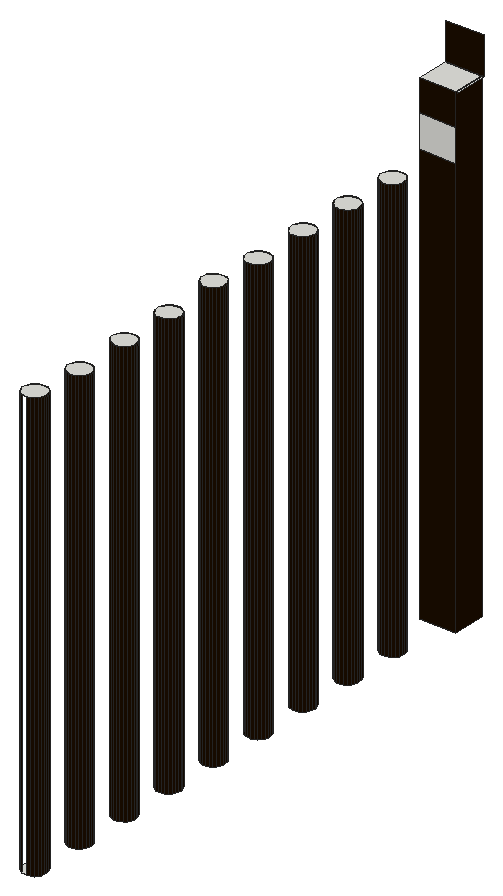
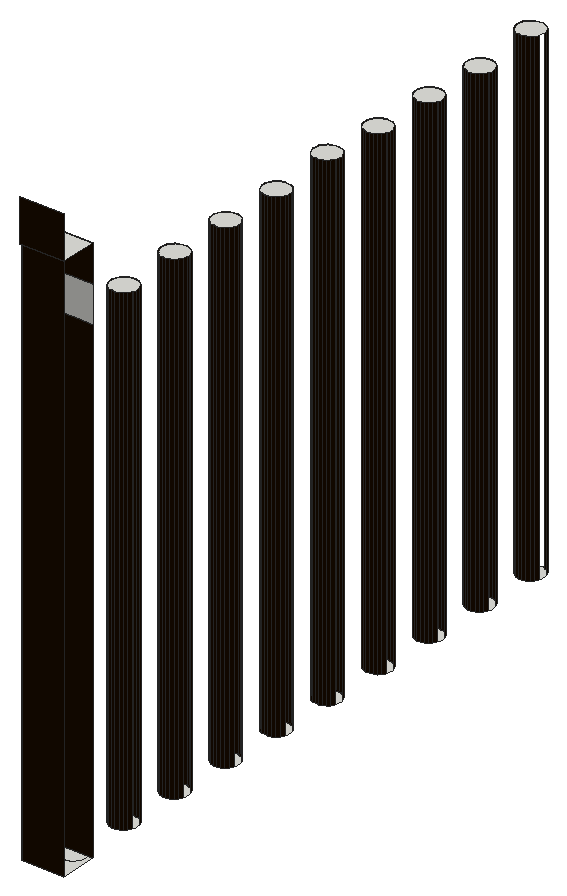
# SketchUp Ruby script. Lengths in inches.
U = 1.inch
M = Sketchup.active_model
def pt(a) = Geom::Point3d.new(a.map { |v| v * U })
def face(e, loops, mat)
  f = e.add_face(loops[0].map { |a| pt(a) })
  loops[1..].each { |l| e.add_face(l.map { |a| pt(a) }).erase! }
  f.material = f.back_material = mat if mat
  f
end
# faces: each face lists its corners as indices into pts; further lists are holes
def faces(e, pts, list, mat = nil) = list.each { |f| face(e, (f[0].is_a?(Array) ? f : [f]).map { |l| l.map { |i| pts[i] } }, mat) }
# xy, xz, yz: faces in a plane at the given z, y or x. An outline is a flat list of corners, or four numbers for a rectangle; further outlines are holes
def ring(l) = l.size == 4 ? [[l[0], l[1]], [l[2], l[1]], [l[2], l[3]], [l[0], l[3]]] : l.each_slice(2).to_a
def flat(e, list, mat, &to3) = list.each { |f| face(e, (f[0].is_a?(Array) ? f : [f]).map { |l| ring(l).map { |u, v| to3.(u, v) } }, mat) }
def xy(e, z, list, mat = nil) = flat(e, list, mat) { |x, y| [x, y, z] }
def xz(e, y, list, mat = nil) = flat(e, list, mat) { |x, z| [x, y, z] }
def yz(e, x, list, mat = nil) = flat(e, list, mat) { |y, z| [x, y, z] }
def lines(e, pts, list) = list.each { |a, b| e.add_line(pt(pts[a]), pt(pts[b])) }
# prism: a flat outline (further loops are holes) pulled along v
def prism(e, loops, v, mat = nil)
  f = face(e, loops, mat); d = Geom::Vector3d.new(v.map { |x| x * U })
  f.pushpull(f.normal.samedirection?(d) ? d.length : -d.length)
end
def box(e, o, s, mat = nil) = prism(e, [[o, [o[0] + s[0], o[1], o[2]], [o[0] + s[0], o[1] + s[1], o[2]], [o[0], o[1] + s[1], o[2]]]], [0, 0, s[2]], mat)
def at(x, y, z, deg = 0) = Geom::Transformation.translation(pt([x, y, z])) * Geom::Transformation.rotation(ORIGIN, Z_AXIS, deg.degrees)
def axes(o, x, y, z) = Geom::Transformation.new([*x, 0, *y, 0, *z, 0, *pt(o).to_a, 1])
def part(name) = M.definitions.add(name)
# library, detail: a bought-in or finely detailed component or shape, given as its bounding box
def library(name, o, s) = part(name).tap { |d| box(d.entities, o, s) }
def detail(e, o, s) = box(e.add_group.entities, o, s)
def put(e, d, t, mat = nil) = e.add_instance(d, t).tap { |i| i.material = mat if mat }
def group(e, t, mat = nil) = e.add_group.tap { |g| g.transformation = t; g.material = mat if mat }.entities
root = M.entities
M.materials.add("[Metal Seamed]1").color = [28, 14, 0]
xy(root,618.25,[[363.55,258.66,363.21,258.75,362.92,258.92,362.67,259.16,362.5,259.46,362.41,259.79,362.41,260.13,362.5,260.46,362.67,260.76,362.91,261,363.2,261.17,363.54,261.26,363.88,261.26,364.21,261.18,364.51,261.01,364.75,260.76,364.92,260.47,365.01,260.14,365.01,259.8,364.93,259.46,364.76,259.17,364.51,258.92,364.22,258.75,363.89,258.66],[363.55,265.1,363.21,265.19,362.92,265.36,362.67,265.6,362.5,265.89,362.41,266.22,362.41,266.57,362.5,266.9,362.67,267.19,362.91,267.4375,363.2,267.61,363.54,267.7,363.88,267.7,364.21,267.61,364.51,267.44,364.75,267.2,364.92,266.91,365.01,266.58,365.01,266.23,364.93,265.9,364.76,265.6,364.51,265.36,364.22,265.1875,363.89,265.1],[363.55,271.54,363.21,271.62,362.92,271.79,362.67,272.03,362.5,272.33,362.41,272.66,362.41,273,362.5,273.33,362.67,273.63,362.91,273.875,363.2,274.05,363.54,274.14,363.88,274.14,364.21,274.05,364.51,273.88,364.75,273.64,364.92,273.34,365.01,273.01,365.01,272.67,364.93,272.34,364.76,272.04,364.51,271.8,364.22,271.625,363.89,271.54],[363.55,277.97,363.21,278.06,362.92,278.23,362.67,278.47,362.5,278.77,362.41,279.1,362.41,279.44,362.5,279.77,362.67,280.07,362.91,280.3125,363.2,280.49,363.54,280.58,363.88,280.58,364.21,280.49,364.51,280.32,364.75,280.08,364.92,279.78,365.01,279.45,365.01,279.11,364.93,278.78,364.76,278.48,364.51,278.24,364.22,278.0625,363.89,277.97],[363.55,284.41,363.21,284.5,362.92,284.67,362.67,284.91,362.5,285.21,362.41,285.54,362.41,285.88,362.5,286.21,362.67,286.51,362.91,286.75,363.2,286.92,363.54,287.01,363.88,287.01,364.21,286.93,364.51,286.76,364.75,286.51,364.92,286.22,365.01,285.89,365.01,285.55,364.93,285.21,364.76,284.92,364.51,284.67,364.22,284.5,363.89,284.41],
  [363.55,290.85,363.21,290.94,362.92,291.11,362.67,291.35,362.5,291.64,362.41,291.97,362.41,292.32,362.5,292.65,362.67,292.94,362.91,293.1875,363.2,293.36,363.54,293.45,363.88,293.45,364.21,293.36,364.51,293.19,364.75,292.95,364.92,292.66,365.01,292.33,365.01,291.98,364.93,291.65,364.76,291.35,364.51,291.11,364.22,290.9375,363.89,290.85],[363.55,297.29,363.21,297.37,362.92,297.54,362.67,297.78,362.5,298.08,362.41,298.41,362.41,298.75,362.5,299.08,362.67,299.38,362.91,299.625,363.2,299.8,363.54,299.89,363.88,299.89,364.21,299.8,364.51,299.63,364.75,299.39,364.92,299.09,365.01,298.76,365.01,298.42,364.93,298.09,364.76,297.79,364.51,297.55,364.22,297.375,363.89,297.29],[363.55,303.72,363.21,303.81,362.92,303.98,362.67,304.22,362.5,304.52,362.41,304.85,362.41,305.19,362.5,305.52,362.67,305.82,362.91,306.0625,363.2,306.24,363.54,306.33,363.88,306.33,364.21,306.24,364.51,306.07,364.75,305.83,364.92,305.53,365.01,305.2,365.01,304.86,364.93,304.53,364.76,304.23,364.51,303.99,364.22,303.8125,363.89,303.72],[363.55,310.16,363.21,310.25,362.92,310.42,362.67,310.66,362.5,310.96,362.41,311.29,362.41,311.63,362.5,311.96,362.67,312.26,362.91,312.5,363.2,312.67,363.54,312.76,363.88,312.76,364.21,312.68,364.51,312.51,364.75,312.26,364.92,311.97,365.01,311.64,365.01,311.3,364.93,310.96,364.76,310.67,364.51,310.42,364.22,310.25,363.89,310.16],[361.98,317.52,361.98,321.28,366.15,321.28,366.15,317.52,364.96,317.52,365.01,317.73,365.01,318.08,364.92,318.41,364.75,318.7,364.51,318.94,364.21,319.11,363.88,319.2,363.54,319.2,363.2,319.11,362.91,318.9375,362.67,318.69,362.5,318.4,362.41,318.07,362.41,317.72,362.47,317.52],
  [362.47,317.52,364.96,317.52,365.01,317.73,365.01,318.08,364.92,318.41,364.75,318.7,364.51,318.94,364.21,319.11,363.88,319.2,363.54,319.2,363.2,319.11,362.91,318.9375,362.67,318.69,362.5,318.4,362.41,318.07,362.41,317.72]])
xy(root,667,[[363.55,310.16,363.89,310.16,364.22,310.25,364.51,310.42,364.76,310.67,364.93,310.96,365.01,311.3,365.01,311.64,364.92,311.97,364.75,312.26,364.51,312.51,364.21,312.68,363.88,312.76,363.54,312.76,363.2,312.67,362.91,312.5,362.67,312.26,362.5,311.96,362.41,311.63,362.41,311.29,362.5,310.96,362.67,310.66,362.92,310.42,363.21,310.25]])
xy(root,667.0625,[[363.55,265.1,363.89,265.1,364.22,265.1875,364.51,265.36,364.76,265.6,364.93,265.9,365.01,266.23,365.01,266.58,364.92,266.91,364.75,267.2,364.51,267.44,364.21,267.61,363.88,267.7,363.54,267.7,363.2,267.61,362.91,267.4375,362.67,267.19,362.5,266.9,362.41,266.57,362.41,266.22,362.5,265.89,362.67,265.6,362.92,265.36,363.21,265.19]])
xy(root,667.1875,[[363.55,290.85,363.89,290.85,364.22,290.9375,364.51,291.11,364.76,291.35,364.93,291.65,365.01,291.98,365.01,292.33,364.92,292.66,364.75,292.95,364.51,293.19,364.21,293.36,363.88,293.45,363.54,293.45,363.2,293.36,362.91,293.1875,362.67,292.94,362.5,292.65,362.41,292.32,362.41,291.97,362.5,291.64,362.67,291.35,362.92,291.11,363.21,290.94],[363.55,303.72,363.89,303.72,364.22,303.8125,364.51,303.99,364.76,304.23,364.93,304.53,365.01,304.86,365.01,305.2,364.92,305.53,364.75,305.83,364.51,306.07,364.21,306.24,363.88,306.33,363.54,306.33,363.2,306.24,362.91,306.0625,362.67,305.82,362.5,305.52,362.41,305.19,362.41,304.85,362.5,304.52,362.67,304.22,362.92,303.98,363.21,303.81]])
xy(root,667.25,[[363.55,271.54,363.89,271.54,364.22,271.625,364.51,271.8,364.76,272.04,364.93,272.34,365.01,272.67,365.01,273.01,364.92,273.34,364.75,273.64,364.51,273.88,364.21,274.05,363.88,274.14,363.54,274.14,363.2,274.05,362.91,273.875,362.67,273.63,362.5,273.33,362.41,273,362.41,272.66,362.5,272.33,362.67,272.03,362.92,271.79,363.21,271.62],[363.55,277.97,363.89,277.97,364.22,278.0625,364.51,278.24,364.76,278.48,364.93,278.78,365.01,279.11,365.01,279.45,364.92,279.78,364.75,280.08,364.51,280.32,364.21,280.49,363.88,280.58,363.54,280.58,363.2,280.49,362.91,280.3125,362.67,280.07,362.5,279.77,362.41,279.44,362.41,279.1,362.5,278.77,362.67,278.47,362.92,278.23,363.21,278.06],[363.55,297.29,363.89,297.29,364.22,297.375,364.51,297.55,364.76,297.79,364.93,298.09,365.01,298.42,365.01,298.76,364.92,299.09,364.75,299.39,364.51,299.63,364.21,299.8,363.88,299.89,363.54,299.89,363.2,299.8,362.91,299.625,362.67,299.38,362.5,299.08,362.41,298.75,362.41,298.41,362.5,298.08,362.67,297.78,362.92,297.54,363.21,297.37]])
xy(root,667.625,[[363.55,258.66,363.89,258.66,364.22,258.75,364.51,258.92,364.76,259.17,364.93,259.46,365.01,259.8,365.01,260.14,364.92,260.47,364.75,260.76,364.51,261.01,364.21,261.18,363.88,261.26,363.54,261.26,363.2,261.17,362.91,261,362.67,260.76,362.5,260.46,362.41,260.13,362.41,259.79,362.5,259.46,362.67,259.16,362.92,258.92,363.21,258.75]])
xy(root,667.6875,[[363.55,284.41,363.89,284.41,364.22,284.5,364.51,284.67,364.76,284.92,364.93,285.21,365.01,285.55,365.01,285.89,364.92,286.22,364.75,286.51,364.51,286.76,364.21,286.93,363.88,287.01,363.54,287.01,363.2,286.92,362.91,286.75,362.67,286.51,362.5,286.21,362.41,285.88,362.41,285.54,362.5,285.21,362.67,284.91,362.92,284.67,363.21,284.5]])
xy(root,674.05,[[361.98,317.52,366.15,321.28],[366.15,317.52,366.34,321.28]])
xz(root,261.26,[[363.54,618.25,363.88,667.625]],"[Metal Seamed]1")
xz(root,265.1,[[363.55,618.25,363.89,667.0625]],"[Metal Seamed]1")
xz(root,267.7,[[363.54,618.25,363.88,667.0625]],"[Metal Seamed]1")
xz(root,271.54,[[363.55,618.25,363.89,667.25]],"[Metal Seamed]1")
xz(root,274.14,[[363.54,618.25,363.88,667.25]],"[Metal Seamed]1")
xz(root,277.97,[[363.55,618.25,363.89,667.25]],"[Metal Seamed]1")
xz(root,280.58,[[363.54,618.25,363.88,667.25]],"[Metal Seamed]1")
xz(root,284.41,[[363.55,618.25,363.89,667.6875]],"[Metal Seamed]1")
xz(root,287.01,[[363.54,618.25,363.88,667.6875]],"[Metal Seamed]1")
xz(root,290.85,[[363.55,618.25,363.89,667.1875]],"[Metal Seamed]1")
xz(root,293.45,[[363.54,618.25,363.88,667.1875]],"[Metal Seamed]1")
xz(root,297.29,[[363.55,618.25,363.89,667.25]],"[Metal Seamed]1")
xz(root,299.89,[[363.54,618.25,363.88,667.25]],"[Metal Seamed]1")
xz(root,303.72,[[363.55,618.25,363.89,667.1875]],"[Metal Seamed]1")
xz(root,306.33,[[363.54,618.25,363.88,667.1875]],"[Metal Seamed]1")
xz(root,310.16,[[363.55,618.25,363.89,667]],"[Metal Seamed]1")
xz(root,312.76,[[363.54,618.25,363.88,667]],"[Metal Seamed]1")
xz(root,317.52,[[361.98,666.66,366.15,670.37]])
xz(root,317.52,[[361.98,618.25,366.15,666.66],[361.98,670.37,366.15,674.05]],"[Metal Seamed]1")
xz(root,321.28,[[361.98,618.25,366.15,674.05],[361.97,674.05,366.34,678.3125]],"[Metal Seamed]1")
yz(root,365.01,[[259.8,618.25,260.14,667.625],[266.23,618.25,266.58,667.0625],[272.67,618.25,273.01,667.25],[279.11,618.25,279.45,667.25],[285.55,618.25,285.89,667.6875],
  [291.98,618.25,292.33,667.1875],[298.42,618.25,298.76,667.25],[304.86,618.25,305.2,667.1875],[311.3,618.25,311.64,667]],"[Metal Seamed]1")
yz(root,366.15,[[317.52,618.25,321.28,674.05]],"[Metal Seamed]1")
p = [[362.92,258.92,618.25],[363.21,258.75,618.25],[363.21,258.75,667.625],[362.92,258.92,667.625],[363.89,258.66,618.25],[364.22,258.75,618.25],
  [364.22,258.75,667.625],[363.89,258.66,667.625],[364.51,258.92,618.25],[364.51,258.92,667.625],[362.67,259.16,618.25],[362.67,259.16,667.625],
  [364.76,259.17,618.25],[364.76,259.17,667.625],[362.5,259.46,618.25],[362.5,259.46,667.625],[364.93,259.46,618.25],[364.93,259.46,667.625],
  [365.01,259.8,618.25],[365.01,259.8,667.625],[365.01,260.14,618.25],[364.92,260.47,618.25],[364.92,260.47,667.625],[365.01,260.14,667.625],
  [362.67,260.76,618.25],[362.5,260.46,618.25],[362.5,260.46,667.625],[362.67,260.76,667.625],[364.75,260.76,618.25],[364.75,260.76,667.625],
  [362.91,261,618.25],[362.91,261,667.625],[364.51,261.01,618.25],[364.51,261.01,667.625],[363.2,261.17,618.25],[363.2,261.17,667.625],
  [364.21,261.18,618.25],[364.21,261.18,667.625],[363.54,261.26,618.25],[363.54,261.26,667.625],[363.88,261.26,618.25],[363.88,261.26,667.625],
  [363.21,265.19,618.25],[363.55,265.1,618.25],[363.55,265.1,667.0625],[363.21,265.19,667.0625],[363.89,265.1,618.25],[364.22,265.1875,618.25],
  [364.22,265.1875,667.0625],[363.89,265.1,667.0625],[362.92,265.36,618.25],[362.92,265.36,667.0625],[364.51,265.36,618.25],[364.51,265.36,667.0625],
  [362.67,265.6,618.25],[362.67,265.6,667.0625],[364.76,265.6,618.25],[364.76,265.6,667.0625],[362.5,265.89,618.25],[362.5,265.89,667.0625],
  [364.93,265.9,618.25],[364.93,265.9,667.0625],[365.01,266.23,618.25],[365.01,266.23,667.0625],[365.01,266.58,618.25],[364.92,266.91,618.25],
  [364.92,266.91,667.0625],[365.01,266.58,667.0625],[362.67,267.19,618.25],[362.5,266.9,618.25],[362.5,266.9,667.0625],[362.67,267.19,667.0625],
  [364.75,267.2,618.25],[364.75,267.2,667.0625],[362.91,267.4375,618.25],[362.91,267.4375,667.0625],[364.51,267.44,618.25],[364.51,267.44,667.0625],
  [363.2,267.61,618.25],[363.2,267.61,667.0625],[364.21,267.61,618.25],[364.21,267.61,667.0625],[363.54,267.7,618.25],[363.54,267.7,667.0625],
  [363.88,267.7,618.25],[363.88,267.7,667.0625],[363.21,271.62,618.25],[363.55,271.54,618.25],[363.55,271.54,667.25],[363.21,271.62,667.25],
  [363.89,271.54,618.25],[364.22,271.625,618.25],[364.22,271.625,667.25],[363.89,271.54,667.25],[362.92,271.79,618.25],[362.92,271.79,667.25],
  [364.51,271.8,618.25],[364.51,271.8,667.25],[362.67,272.03,618.25],[362.67,272.03,667.25],[364.76,272.04,618.25],[364.76,272.04,667.25],
  [362.5,272.33,618.25],[362.5,272.33,667.25],[364.93,272.34,618.25],[364.93,272.34,667.25],[365.01,272.67,618.25],[365.01,272.67,667.25],
  [365.01,273.01,618.25],[364.92,273.34,618.25],[364.92,273.34,667.25],[365.01,273.01,667.25],[362.67,273.63,618.25],[362.5,273.33,618.25],
  [362.5,273.33,667.25],[362.67,273.63,667.25],[364.75,273.64,618.25],[364.75,273.64,667.25],[362.91,273.875,618.25],[362.91,273.875,667.25],
  [364.51,273.88,618.25],[364.51,273.88,667.25],[363.2,274.05,618.25],[363.2,274.05,667.25],[364.21,274.05,618.25],[364.21,274.05,667.25],
  [363.54,274.14,618.25],[363.54,274.14,667.25],[363.88,274.14,618.25],[363.88,274.14,667.25],[363.21,278.06,618.25],[363.55,277.97,618.25],
  [363.55,277.97,667.25],[363.21,278.06,667.25],[363.89,277.97,618.25],[364.22,278.0625,618.25],[364.22,278.0625,667.25],[363.89,277.97,667.25],
  [362.92,278.23,618.25],[362.92,278.23,667.25],[364.51,278.24,618.25],[364.51,278.24,667.25],[362.67,278.47,618.25],[362.67,278.47,667.25],
  [364.76,278.48,618.25],[364.76,278.48,667.25],[362.5,278.77,618.25],[362.5,278.77,667.25],[364.93,278.78,618.25],[364.93,278.78,667.25],
  [365.01,279.11,618.25],[365.01,279.11,667.25],[365.01,279.45,618.25],[364.92,279.78,618.25],[364.92,279.78,667.25],[365.01,279.45,667.25],
  [362.67,280.07,618.25],[362.5,279.77,618.25],[362.5,279.77,667.25],[362.67,280.07,667.25],[364.75,280.08,618.25],[364.75,280.08,667.25],
  [362.91,280.3125,618.25],[362.91,280.3125,667.25],[364.51,280.32,618.25],[364.51,280.32,667.25],[363.2,280.49,618.25],[363.2,280.49,667.25],
  [364.21,280.49,618.25],[364.21,280.49,667.25],[363.54,280.58,618.25],[363.54,280.58,667.25],[363.88,280.58,618.25],[363.88,280.58,667.25],
  [363.21,284.5,618.25],[363.55,284.41,618.25],[363.55,284.41,667.6875],[363.21,284.5,667.6875],[363.89,284.41,618.25],[364.22,284.5,618.25],
  [364.22,284.5,667.6875],[363.89,284.41,667.6875],[362.92,284.67,618.25],[362.92,284.67,667.6875],[364.51,284.67,618.25],[364.51,284.67,667.6875],
  [362.67,284.91,618.25],[362.67,284.91,667.6875],[364.76,284.92,618.25],[364.76,284.92,667.6875],[362.5,285.21,618.25],[362.5,285.21,667.6875],
  [364.93,285.21,618.25],[364.93,285.21,667.6875],[365.01,285.55,618.25],[365.01,285.55,667.6875],[365.01,285.89,618.25],[364.92,286.22,618.25],
  [364.92,286.22,667.6875],[365.01,285.89,667.6875],[362.67,286.51,618.25],[362.5,286.21,618.25],[362.5,286.21,667.6875],[362.67,286.51,667.6875],
  [364.75,286.51,618.25],[364.75,286.51,667.6875],[362.91,286.75,618.25],[362.91,286.75,667.6875],[364.51,286.76,618.25],[364.51,286.76,667.6875],
  [363.2,286.92,618.25],[363.2,286.92,667.6875],[364.21,286.93,618.25],[364.21,286.93,667.6875],[363.54,287.01,618.25],[363.54,287.01,667.6875],
  [363.88,287.01,618.25],[363.88,287.01,667.6875],[363.21,290.94,618.25],[363.55,290.85,618.25],[363.55,290.85,667.1875],[363.21,290.94,667.1875],
  [363.89,290.85,618.25],[364.22,290.9375,618.25],[364.22,290.9375,667.1875],[363.89,290.85,667.1875],[362.92,291.11,618.25],[362.92,291.11,667.1875],
  [364.51,291.11,618.25],[364.51,291.11,667.1875],[362.67,291.35,618.25],[362.67,291.35,667.1875],[364.76,291.35,618.25],[364.76,291.35,667.1875],
  [362.5,291.64,618.25],[362.5,291.64,667.1875],[364.93,291.65,618.25],[364.93,291.65,667.1875],[365.01,291.98,618.25],[365.01,291.98,667.1875],
  [365.01,292.33,618.25],[364.92,292.66,618.25],[364.92,292.66,667.1875],[365.01,292.33,667.1875],[362.67,292.94,618.25],[362.5,292.65,618.25],
  [362.5,292.65,667.1875],[362.67,292.94,667.1875],[364.75,292.95,618.25],[364.75,292.95,667.1875],[362.91,293.1875,618.25],[362.91,293.1875,667.1875],
  [364.51,293.19,618.25],[364.51,293.19,667.1875],[363.2,293.36,618.25],[363.2,293.36,667.1875],[364.21,293.36,618.25],[364.21,293.36,667.1875],
  [363.54,293.45,618.25],[363.54,293.45,667.1875],[363.88,293.45,618.25],[363.88,293.45,667.1875],[363.21,297.37,618.25],[363.55,297.29,618.25],
  [363.55,297.29,667.25],[363.21,297.37,667.25],[363.89,297.29,618.25],[364.22,297.375,618.25],[364.22,297.375,667.25],[363.89,297.29,667.25],
  [362.92,297.54,618.25],[362.92,297.54,667.25],[364.51,297.55,618.25],[364.51,297.55,667.25],[362.67,297.78,618.25],[362.67,297.78,667.25],
  [364.76,297.79,618.25],[364.76,297.79,667.25],[362.5,298.08,618.25],[362.5,298.08,667.25],[364.93,298.09,618.25],[364.93,298.09,667.25],
  [365.01,298.42,618.25],[365.01,298.42,667.25],[365.01,298.76,618.25],[364.92,299.09,618.25],[364.92,299.09,667.25],[365.01,298.76,667.25],
  [362.67,299.38,618.25],[362.5,299.08,618.25],[362.5,299.08,667.25],[362.67,299.38,667.25],[364.75,299.39,618.25],[364.75,299.39,667.25],
  [362.91,299.625,618.25],[362.91,299.625,667.25],[364.51,299.63,618.25],[364.51,299.63,667.25],[363.2,299.8,618.25],[363.2,299.8,667.25],
  [364.21,299.8,618.25],[364.21,299.8,667.25],[363.54,299.89,618.25],[363.54,299.89,667.25],[363.88,299.89,618.25],[363.88,299.89,667.25],
  [363.21,303.81,618.25],[363.55,303.72,618.25],[363.55,303.72,667.1875],[363.21,303.81,667.1875],[363.89,303.72,618.25],[364.22,303.8125,618.25],
  [364.22,303.8125,667.1875],[363.89,303.72,667.1875],[362.92,303.98,618.25],[362.92,303.98,667.1875],[364.51,303.99,618.25],[364.51,303.99,667.1875],
  [362.67,304.22,618.25],[362.67,304.22,667.1875],[364.76,304.23,618.25],[364.76,304.23,667.1875],[362.5,304.52,618.25],[362.5,304.52,667.1875],
  [364.93,304.53,618.25],[364.93,304.53,667.1875],[365.01,304.86,618.25],[365.01,304.86,667.1875],[365.01,305.2,618.25],[364.92,305.53,618.25],
  [364.92,305.53,667.1875],[365.01,305.2,667.1875],[362.67,305.82,618.25],[362.5,305.52,618.25],[362.5,305.52,667.1875],[362.67,305.82,667.1875],
  [364.75,305.83,618.25],[364.75,305.83,667.1875],[362.91,306.0625,618.25],[362.91,306.0625,667.1875],[364.51,306.07,618.25],[364.51,306.07,667.1875],
  [363.2,306.24,618.25],[363.2,306.24,667.1875],[364.21,306.24,618.25],[364.21,306.24,667.1875],[363.54,306.33,618.25],[363.54,306.33,667.1875],
  [363.88,306.33,618.25],[363.88,306.33,667.1875],[362.92,310.42,618.25],[363.21,310.25,618.25],[363.21,310.25,667],[362.92,310.42,667],
  [363.55,310.16,618.25],[363.55,310.16,667],[363.89,310.16,618.25],[364.22,310.25,618.25],[364.22,310.25,667],[363.89,310.16,667],
  [364.51,310.42,618.25],[364.51,310.42,667],[362.67,310.66,618.25],[362.67,310.66,667],[364.76,310.67,618.25],[364.76,310.67,667],
  [362.5,310.96,618.25],[362.5,310.96,667],[364.93,310.96,618.25],[364.93,310.96,667],[365.01,311.3,618.25],[365.01,311.3,667],
  [365.01,311.64,618.25],[364.92,311.97,618.25],[364.92,311.97,667],[365.01,311.64,667],[362.67,312.26,618.25],[362.5,311.96,618.25],
  [362.5,311.96,667],[362.67,312.26,667],[364.75,312.26,618.25],[364.75,312.26,667],[362.91,312.5,618.25],[362.91,312.5,667],
  [364.51,312.51,618.25],[364.51,312.51,667],[363.2,312.67,618.25],[363.2,312.67,667],[364.21,312.68,618.25],[364.21,312.68,667],
  [363.54,312.76,618.25],[363.54,312.76,667],[363.88,312.76,618.25],[363.88,312.76,667],[366.15,317.52,674.375],[366.15,317.52,674.05],
  [366.34,317.52,674.375]]
faces(root,p,[[0,1,2,3],[4,5,6,7],[5,8,9,6],[10,0,3,11],[8,12,13,9],[14,10,11,15],[12,16,17,13],[16,18,19,17],
  [20,21,22,23],[24,25,26,27],[21,28,29,22],[30,24,27,31],[28,32,33,29],[34,30,31,35],[32,36,37,33],[38,34,35,39],
  [36,40,41,37],[42,43,44,45],[46,47,48,49],[50,42,45,51],[47,52,53,48],[54,50,51,55],[52,56,57,53],[58,54,55,59],
  [56,60,61,57],[60,62,63,61],[64,65,66,67],[68,69,70,71],[65,72,73,66],[74,68,71,75],[72,76,77,73],[78,74,75,79],
  [76,80,81,77],[82,78,79,83],[80,84,85,81],[86,87,88,89],[90,91,92,93],[94,86,89,95],[91,96,97,92],[98,94,95,99],
  [96,100,101,97],[102,98,99,103],[100,104,105,101],[104,106,107,105],[108,109,110,111],[112,113,114,115],[109,116,117,110],[118,112,115,119],
  [116,120,121,117],[122,118,119,123],[120,124,125,121],[126,122,123,127],[124,128,129,125],[130,131,132,133],[134,135,136,137],[138,130,133,139],
  [135,140,141,136],[142,138,139,143],[140,144,145,141],[146,142,143,147],[144,148,149,145],[148,150,151,149],[152,153,154,155],[156,157,158,159],
  [153,160,161,154],[162,156,159,163],[160,164,165,161],[166,162,163,167],[164,168,169,165],[170,166,167,171],[168,172,173,169],[174,175,176,177],
  [178,179,180,181],[182,174,177,183],[179,184,185,180],[186,182,183,187],[184,188,189,185],[190,186,187,191],[188,192,193,189],[192,194,195,193],
  [196,197,198,199],[200,201,202,203],[197,204,205,198],[206,200,203,207],[204,208,209,205],[210,206,207,211],[208,212,213,209],[214,210,211,215],
  [212,216,217,213],[218,219,220,221],[222,223,224,225],[226,218,221,227],[223,228,229,224],[230,226,227,231],[228,232,233,229],[234,230,231,235],
  [232,236,237,233],[236,238,239,237],[240,241,242,243],[244,245,246,247],[241,248,249,242],[250,244,247,251],[248,252,253,249],[254,250,251,255],
  [252,256,257,253],[258,254,255,259],[256,260,261,257],[262,263,264,265],[266,267,268,269],[270,262,265,271],[267,272,273,268],[274,270,271,275],
  [272,276,277,273],[278,274,275,279],[276,280,281,277],[280,282,283,281],[284,285,286,287],[288,289,290,291],[285,292,293,286],[294,288,291,295],
  [292,296,297,293],[298,294,295,299],[296,300,301,297],[302,298,299,303],[300,304,305,301],[306,307,308,309],[310,311,312,313],[314,306,309,315],
  [311,316,317,312],[318,314,315,319],[316,320,321,317],[322,318,319,323],[320,324,325,321],[324,326,327,325],[328,329,330,331],[332,333,334,335],
  [329,336,337,330],[338,332,335,339],[336,340,341,337],[342,338,339,343],[340,344,345,341],[346,342,343,347],[344,348,349,345],[350,351,352,353],
  [351,354,355,352],[356,357,358,359],[357,360,361,358],[362,350,353,363],[360,364,365,361],[366,362,363,367],[364,368,369,365],[368,370,371,369],
  [372,373,374,375],[376,377,378,379],[373,380,381,374],[382,376,379,383],[380,384,385,381],[386,382,383,387],[384,388,389,385],[390,386,387,391],
  [388,392,393,389]],"[Metal Seamed]1")
lines(root,p,[[394,395],[394,396]])
